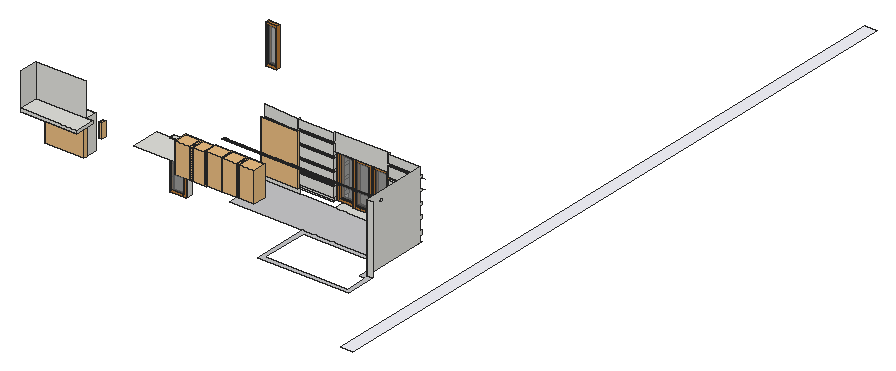
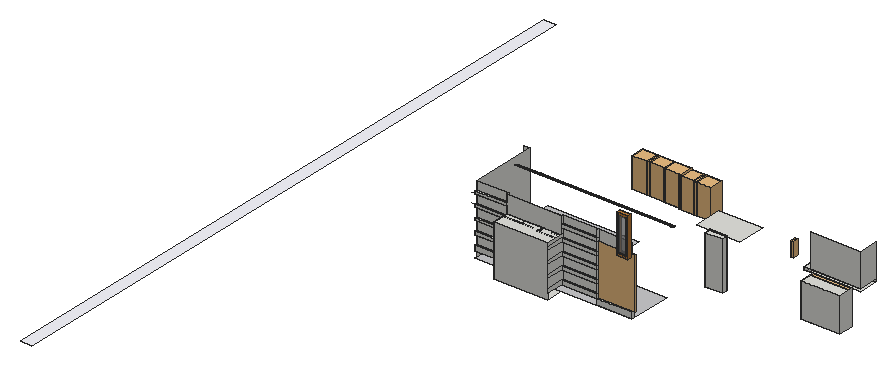
# SketchUp Ruby script. Lengths in inches.
U = 1.inch
M = Sketchup.active_model
def pt(a) = Geom::Point3d.new(a.map { |v| v * U })
def face(e, loops, mat)
  f = e.add_face(loops[0].map { |a| pt(a) })
  loops[1..].each { |l| e.add_face(l.map { |a| pt(a) }).erase! }
  f.material = f.back_material = mat if mat
  f
end
# faces: each face lists its corners as indices into pts; further lists are holes
def faces(e, pts, list, mat = nil) = list.each { |f| face(e, (f[0].is_a?(Array) ? f : [f]).map { |l| l.map { |i| pts[i] } }, mat) }
# xy, xz, yz: faces in a plane at the given z, y or x. An outline is a flat list of corners, or four numbers for a rectangle; further outlines are holes
def ring(l) = l.size == 4 ? [[l[0], l[1]], [l[2], l[1]], [l[2], l[3]], [l[0], l[3]]] : l.each_slice(2).to_a
def flat(e, list, mat, &to3) = list.each { |f| face(e, (f[0].is_a?(Array) ? f : [f]).map { |l| ring(l).map { |u, v| to3.(u, v) } }, mat) }
def xy(e, z, list, mat = nil) = flat(e, list, mat) { |x, y| [x, y, z] }
def xz(e, y, list, mat = nil) = flat(e, list, mat) { |x, z| [x, y, z] }
def yz(e, x, list, mat = nil) = flat(e, list, mat) { |y, z| [x, y, z] }
def lines(e, pts, list) = list.each { |a, b| e.add_line(pt(pts[a]), pt(pts[b])) }
# prism: a flat outline (further loops are holes) pulled along v
def prism(e, loops, v, mat = nil)
  f = face(e, loops, mat); d = Geom::Vector3d.new(v.map { |x| x * U })
  f.pushpull(f.normal.samedirection?(d) ? d.length : -d.length)
end
def box(e, o, s, mat = nil) = prism(e, [[o, [o[0] + s[0], o[1], o[2]], [o[0] + s[0], o[1] + s[1], o[2]], [o[0], o[1] + s[1], o[2]]]], [0, 0, s[2]], mat)
def at(x, y, z, deg = 0) = Geom::Transformation.translation(pt([x, y, z])) * Geom::Transformation.rotation(ORIGIN, Z_AXIS, deg.degrees)
def axes(o, x, y, z) = Geom::Transformation.new([*x, 0, *y, 0, *z, 0, *pt(o).to_a, 1])
def part(name) = M.definitions.add(name)
# library, detail: a bought-in or finely detailed component or shape, given as its bounding box
def library(name, o, s) = part(name).tap { |d| box(d.entities, o, s) }
def detail(e, o, s) = box(e.add_group.entities, o, s)
def put(e, d, t, mat = nil) = e.add_instance(d, t).tap { |i| i.material = mat if mat }
def group(e, t, mat = nil) = e.add_group.tap { |g| g.transformation = t; g.material = mat if mat }.entities
root = M.entities
M.materials.add("TEAKcrown-cut").color = [186, 122, 55]
M.materials.add("[0117_GhostWhite]").color = [248, 248, 255]
M.materials.add("[Polished Concrete New]").color = [200, 200, 203]
M.materials.add("[Translucent_Glass_Gray]").color = [128, 128, 128]
M.materials["[Translucent_Glass_Gray]"].alpha = 0.5
c1 = part("Senza")
g1 = group(c1.entities,at(-137.05,828.91,-82.14))
detail(g1,[0,0,0],[37.72,1.46,81.14])
c2 = part("Group\#4")
xy(c2.entities,0,[[0,0,17.12,1]],"TEAKcrown-cut")
xy(c2.entities,2.5,[[2.5,0,14.62,0.4],[2.5,0.6,14.62,1]],"TEAKcrown-cut")
xy(c2.entities,2.5,[[2.5,0.4,14.62,0.6]],"[Translucent_Glass_Gray]")
xy(c2.entities,46.29,[[2.5,0,14.62,0.4],[2.5,0.6,14.62,1]],"TEAKcrown-cut")
xy(c2.entities,46.29,[[2.5,0.4,14.62,0.6]],"[Translucent_Glass_Gray]")
xy(c2.entities,48.79,[[0,0,17.12,1]],"TEAKcrown-cut")
xz(c2.entities,0,[[[0,0,17.12,48.79],[2.5,2.5,14.62,46.29]]],"TEAKcrown-cut")
xz(c2.entities,0.4,[[2.5,2.5,14.62,46.29]],"[Translucent_Glass_Gray]")
xz(c2.entities,0.6,[[2.5,2.5,14.62,46.29]],"[Translucent_Glass_Gray]")
xz(c2.entities,1,[[[0,0,17.12,48.79],[2.5,2.5,14.62,46.29]]],"TEAKcrown-cut")
yz(c2.entities,0,[[0,0,1,48.79]],"TEAKcrown-cut")
yz(c2.entities,2.5,[[0,2.5,0.4,46.29],[0.6,2.5,1,46.29]],"TEAKcrown-cut")
yz(c2.entities,2.5,[[0.4,2.5,0.6,46.29]],"[Translucent_Glass_Gray]")
yz(c2.entities,14.62,[[0,2.5,0.4,46.29],[0.6,2.5,1,46.29]],"TEAKcrown-cut")
yz(c2.entities,14.62,[[0.4,2.5,0.6,46.29]],"[Translucent_Glass_Gray]")
yz(c2.entities,17.12,[[0,0,1,48.79]],"TEAKcrown-cut")
c3 = part("window\#1")
p = [[34.85,2.5,83],[34.85,-1.5,83]]
lines(c3.entities,p,[[0,1]])
put(c3.entities,c2,axes([57.69,622.6,-63.625],[2.8784,0,0],[0,2.8784,0],[0,0,2.8784]))
g2 = group(c3.entities,at(372.25,848.48,-68.54))
put(g2,c2,axes([49.78,-5.16,0],[3.10271,0,0],[0,-14.14627,0],[0,0,2.62942]))
put(g2,c2,axes([102.89,-5.16,0],[3.10271,0,0],[0,-14.14627,0],[0,0,2.62942]))
put(g2,c2,axes([0,0,0],[3.10271,0,0],[0,-14.14627,0],[0,0,2.62942]))
put(c3.entities,c2,axes([93.6875,937.15,140.85],[1.86518,0,0],[0,-10.84408,0],[0,0,2.32063]))
c4 = library("window\#2",[0,0,0],[78.15,10.2,70.87])
c5 = library("Thorburn+Narrow+Wall+Sconce+-+Dark+Aluminum",[0,-1.5,-7.55],[4.87,3,15.1])
c6 = library("climbing plant",[8874.76,-5589.78,-33.625],[50.13,38.07,87.16])
xy(root,29.3125,[[1176.26,719.78,1299.63,769.53],[1299.63,719.78,1332.64,769.53]])
xy(root,29.3125,[[[1182.84,433.09,1443.95,433.09,1443.95,521.59,1425.51,521.59,1425.51,594.47,1182.84,594.47],[1193.75,444.01,1193.75,583.56,1414.59,583.56,1414.59,510.68,1433.03,510.68,1433.03,444.01]],[971.9,594.47,1425.51,719.78]],"[Polished Concrete New]")
xy(root,46.83,[[1332.64,714.35,1425.51,719.78]])
xy(root,46.92,[[1074.08,714.35,1074.08,719.78,971.9,719.78],[971.9,714.35,1074.08,714.35,971.9,719.78],[1074.08,714.35,1176.26,719.78]])
xy(root,51.84,[[862.83,515.34,912.07,531.28]])
xy(root,57.97,[[1074.08,714.35,1176.26,719.78]])
xy(root,61.06,[[1332.64,714.35,1425.51,719.78]])
xy(root,67.73,[[522.65,490.53,633.9,534.03]])
xy(root,85.73,[[1074.08,714.35,1176.26,719.78]])
xy(root,88.83,[[1332.64,714.35,1425.51,719.78]])
xy(root,94.16,[[1074.08,714.35,1176.26,719.78]])
xy(root,97.88,[[1332.64,714.35,1425.51,719.78]])
xy(root,121.92,[[1074.08,714.35,1176.26,719.78]])
xy(root,125.64,[[1332.64,714.35,1425.51,719.78]])
xy(root,130.35,[[1074.08,714.35,1176.26,719.78]])
xy(root,132.44,[[1332.64,714.35,1425.51,719.78]])
xy(root,158.11,[[1074.08,714.35,1176.26,719.78]])
xy(root,160.2,[[1332.64,714.35,1425.51,719.78]])
xy(root,166.1,[[497.32,433.09,497.32,490.53,522.65,490.53,522.65,534.03,633.9,534.03,633.9,490.53,660.32,490.53,660.32,433.09]])
xy(root,166.54,[[1074.08,714.35,1176.26,719.78]])
xy(root,167.19,[[1332.64,714.35,1425.51,719.78]])
xy(root,174.17,[[497.32,433.09,660.32,490.53]])
xy(root,175.27,[[1176.26,719.78,1332.64,769.53]])
xy(root,191.73,[[825.44,433.09,825.44,515.34,862.83,515.34,862.83,531.28,912.07,531.28,912.07,515.34,950.63,515.34,950.63,433.09]])
xy(root,193.9375,[[1769.06,0,1802.44,1887.6875]],"[0117_GhostWhite]")
xy(root,194.3,[[1074.08,714.35,1176.26,719.78]])
xy(root,194.95,[[1332.64,714.35,1425.51,719.78]])
xy(root,202.53,[[1361.93,564.77,1362.51,564.88,1363.04,565.14,1363.48,565.52,1363.8125,566.01,1364,566.5625,1364.05,567.15,1363.94,567.72,1363.68,568.25,1363.3,568.69,1362.8125,569.02,1362.26,569.22,1361.67,569.26,1361.1,569.15,1360.57,568.89,1360.125,568.51,1359.8,568.02,1359.6,567.47,1359.5625,566.88,1359.67,566.31,1359.93,565.78,1360.3125,565.34,1360.8,565.01,1361.35,564.82],[1332.64,714.35,1425.51,719.78]])
xy(root,202.78,[[1074.08,714.35,1176.26,719.78]])
xz(root,433.09,[[497.32,166.1,660.32,174.17]])
xz(root,490.53,[[640.85,166.1,660.32,174.17],[497.32,174.17,640.85,269.5625]])
xz(root,521.59,[[1425.51,29.3125,1443.95,225.29]])
xz(root,531.28,[[862.83,51.84,912.07,191.73]])
xz(root,534.03,[[522.65,67.73,633.9,166.1]])
xz(root,714.35,[[1074.08,57.97,1176.26,85.73],[1332.64,61.06,1425.51,88.83],[1074.08,94.16,1176.26,121.92],[1332.64,97.88,1425.51,125.64],[1074.08,130.35,1176.26,158.11],
  [1332.64,132.44,1425.51,160.2],[1074.08,166.54,1176.26,194.3],[1332.64,167.19,1425.51,194.95],[1332.64,202.53,1425.51,225.29],[1074.08,202.78,1176.26,225.29]])
xz(root,719.78,[[971.9,29.3125,1074.08,46.92],[1332.64,46.83,1425.51,61.06],[1074.08,46.92,1176.26,57.97],[1074.08,85.73,1176.26,94.16],[1332.64,88.83,1425.51,97.88],
  [1074.08,121.92,1176.26,130.35],[1332.64,125.64,1425.51,132.44],[1074.08,158.11,1176.26,166.54],[1332.64,160.2,1425.51,167.19],[1176.26,175.27,1332.64,225.29],
  [1074.08,194.3,1176.26,202.78],[1332.64,194.95,1425.51,202.53]])
xz(root,769.53,[[1176.26,29.3125,1332.64,175.27]])
yz(root,497.32,[[433.09,174.17,490.53,269.5625]])
yz(root,522.65,[[490.53,67.73,534.03,166.1]])
yz(root,633.9,[[490.53,67.73,534.03,166.1]])
yz(root,660.32,[[433.09,166.1,490.53,174.17]])
yz(root,862.83,[[515.34,51.84,531.28,191.73]])
yz(root,912.07,[[515.34,51.84,531.28,191.73]])
yz(root,971.9,[[714.35,29.3125,719.78,46.92]])
yz(root,1074.08,[[714.35,46.92,719.78,57.97],[714.35,57.97,719.78,85.73],[714.35,85.73,719.78,94.16],[714.35,94.16,719.78,121.92],[714.35,121.92,719.78,130.35],
  [714.35,130.35,719.78,158.11],[714.35,158.11,719.78,166.54],[714.35,166.54,719.78,194.3],[714.35,194.3,719.78,202.78],[714.35,202.78,719.78,225.29]])
yz(root,1176.26,[[719.78,46.92,769.53,57.97],[714.35,57.97,769.53,85.73],[719.78,85.73,769.53,94.16],[714.35,94.16,769.53,121.92],[719.78,121.92,769.53,130.35],
  [714.35,130.35,769.53,158.11],[719.78,158.11,769.53,166.54],[714.35,166.54,769.53,175.27],[714.35,175.27,719.78,194.3],[714.35,202.78,719.78,225.29]])
yz(root,1332.64,[[719.78,29.3125,769.53,46.83],[719.78,46.83,769.53,46.92],[719.78,46.92,769.53,61.06],[714.35,61.06,769.53,88.83],[719.78,88.83,769.53,97.88],
  [714.35,97.88,769.53,125.64],[719.78,125.64,769.53,132.44],[714.35,132.44,769.53,160.2],[719.78,160.2,769.53,167.19],[714.35,167.19,769.53,169.59],
  [714.35,169.59,769.53,175.27],[714.35,175.27,719.78,194.95],[714.35,202.53,719.78,225.29]])
yz(root,1425.51,[[521.59,29.3125,521.59,225.29,714.35,225.29,714.35,202.53,719.78,202.53,719.78,194.95,714.35,194.95,714.35,167.19,719.78,167.19,719.78,160.2,714.35,160.2,714.35,132.44,719.78,132.44,719.78,125.64,714.35,125.64,714.35,97.88,719.78,97.88,719.78,88.83,714.35,88.83,714.35,61.06,719.78,61.06,719.78,46.83,714.35,46.83,714.35,29.3125]])
yz(root,1428.71,[[569.58,201.42,570.24,201.51,570.86,201.76,571.39,202.17,571.8,202.7,572.05,203.32,572.14,203.98,572.05,204.64,571.8,205.26,571.39,205.79,570.86,206.2,570.24,206.46,569.58,206.54,568.92,206.46,568.3,206.2,567.77,205.79,567.36,205.26,567.1,204.64,567.02,203.98,567.1,203.32,567.36,202.7,567.77,202.17,568.3,201.76,568.92,201.51]])
p = [[971.9,719.78,225.29],[971.9,719.78,194.3],[1074.08,714.35,194.3],[1074.08,714.35,202.78],[1074.08,714.35,225.29],[971.9,568.92,201.51],
  [971.9,569.58,201.42],[1428.71,569.58,201.42],[1428.71,568.92,201.51],[971.9,570.24,201.51],[1428.71,570.24,201.51],[971.9,568.3,201.76],
  [1428.71,568.3,201.76],[971.9,570.86,201.76],[1428.71,570.86,201.76],[971.9,567.77,202.17],[1428.71,567.77,202.17],[971.9,571.39,202.17],
  [1428.71,571.39,202.17],[971.9,567.36,202.7],[1428.71,567.36,202.7],[971.9,571.8,202.7],[1428.71,571.8,202.7],[971.9,567.1,203.32],
  [1428.71,567.1,203.32],[971.9,572.05,203.32],[1428.71,572.05,203.32],[971.9,567.02,203.98],[1428.71,567.02,203.98],[1361.8,567.02,203.98],
  [971.9,572.14,203.98],[983.58,572.14,203.98],[988.82,572.14,203.98],[1028.52,572.14,203.98],[1033.75,572.14,203.98],[1073.46,572.14,203.98],
  [1078.69,572.14,203.98],[1118.39,572.14,203.98],[1123.63,572.14,203.98],[1163.33,572.14,203.98],[1168.57,572.14,203.98],[1208.27,572.14,203.98],
  [1213.5,572.14,203.98],[1253.21,572.14,203.98],[1258.44,572.14,203.98],[1298.14,572.14,203.98],[1303.38,572.14,203.98],[1343.08,572.14,203.98],
  [1348.32,572.14,203.98],[1388.02,572.14,203.98],[1393.25,572.14,203.98],[1428.71,572.14,203.98],[1434.83,719.78,194.95],[1425.51,719.78,194.95],
  [1425.51,719.78,167.19],[1434.83,719.78,167.19]]
faces(root,p,[[0,1,2,3,4],[5,6,7,8],[6,9,10,7],[11,5,8,12],[9,13,14,10],[15,11,12,16],[13,17,18,14],[19,15,16,20],
  [17,21,22,18],[23,19,20,24],[21,25,26,22],[27,23,24,28,29],[25,30,31,32,33,34,35,36,37,38,39,40,41,42,43,44,45,46,47,48,49,50,51,26]])
lines(root,p,[[52,53],[54,55]])
put(root,c1,axes([1352.23,-788.18,195.58],[2.80009,0,0],[0,1.81,0],[0,0,1.81]))
put(root,c3,at(805.13,-109.13,115.46))
put(root,c4,axes([522.65,490.53,67.73],[1.42355,0,0],[0,1,0],[0,0,1.38818]))
put(root,c5,axes([716.38,461.15,186.64],[0,-2.73,0],[2.73,0,0],[0,0,2.73]))
put(root,c6,at(-7917.98,6006.88,205.16))
put(root,c6,at(-7876.42,6006.88,205.16))
put(root,c6,at(-7832.61,6006.88,208.16))
put(root,c6,at(-7741.42,6006.88,208.16))
put(root,c6,at(-7784.17,6006.88,208.16))
